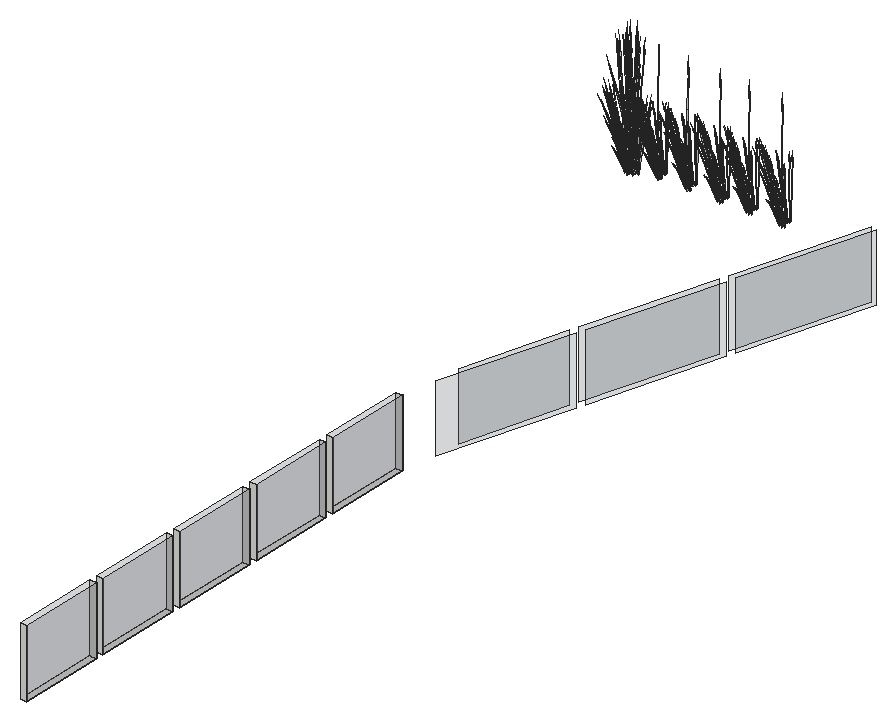
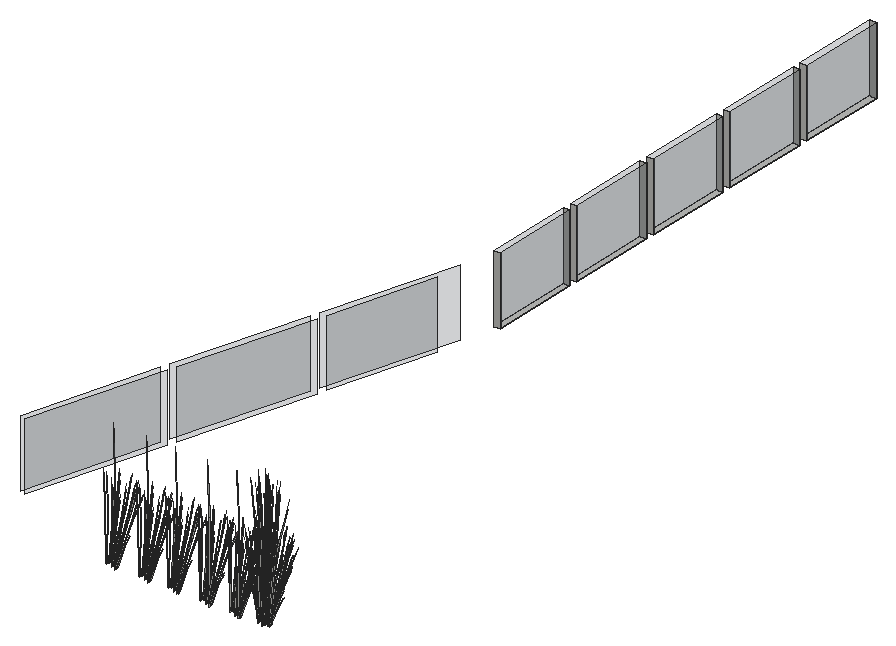
# SketchUp Ruby script. Lengths in inches.
U = 1.inch
M = Sketchup.active_model
def pt(a) = Geom::Point3d.new(a.map { |v| v * U })
def face(e, loops, mat)
  f = e.add_face(loops[0].map { |a| pt(a) })
  loops[1..].each { |l| e.add_face(l.map { |a| pt(a) }).erase! }
  f.material = f.back_material = mat if mat
  f
end
# faces: each face lists its corners as indices into pts; further lists are holes
def faces(e, pts, list, mat = nil) = list.each { |f| face(e, (f[0].is_a?(Array) ? f : [f]).map { |l| l.map { |i| pts[i] } }, mat) }
# xy, xz, yz: faces in a plane at the given z, y or x. An outline is a flat list of corners, or four numbers for a rectangle; further outlines are holes
def ring(l) = l.size == 4 ? [[l[0], l[1]], [l[2], l[1]], [l[2], l[3]], [l[0], l[3]]] : l.each_slice(2).to_a
def flat(e, list, mat, &to3) = list.each { |f| face(e, (f[0].is_a?(Array) ? f : [f]).map { |l| ring(l).map { |u, v| to3.(u, v) } }, mat) }
def xy(e, z, list, mat = nil) = flat(e, list, mat) { |x, y| [x, y, z] }
def xz(e, y, list, mat = nil) = flat(e, list, mat) { |x, z| [x, y, z] }
def yz(e, x, list, mat = nil) = flat(e, list, mat) { |y, z| [x, y, z] }
def lines(e, pts, list) = list.each { |a, b| e.add_line(pt(pts[a]), pt(pts[b])) }
# prism: a flat outline (further loops are holes) pulled along v
def prism(e, loops, v, mat = nil)
  f = face(e, loops, mat); d = Geom::Vector3d.new(v.map { |x| x * U })
  f.pushpull(f.normal.samedirection?(d) ? d.length : -d.length)
end
def box(e, o, s, mat = nil) = prism(e, [[o, [o[0] + s[0], o[1], o[2]], [o[0] + s[0], o[1] + s[1], o[2]], [o[0], o[1] + s[1], o[2]]]], [0, 0, s[2]], mat)
def at(x, y, z, deg = 0) = Geom::Transformation.translation(pt([x, y, z])) * Geom::Transformation.rotation(ORIGIN, Z_AXIS, deg.degrees)
def axes(o, x, y, z) = Geom::Transformation.new([*x, 0, *y, 0, *z, 0, *pt(o).to_a, 1])
def part(name) = M.definitions.add(name)
# library, detail: a bought-in or finely detailed component or shape, given as its bounding box
def library(name, o, s) = part(name).tap { |d| box(d.entities, o, s) }
def detail(e, o, s) = box(e.add_group.entities, o, s)
def put(e, d, t, mat = nil) = e.add_instance(d, t).tap { |i| i.material = mat if mat }
def group(e, t, mat = nil) = e.add_group.tap { |g| g.transformation = t; g.material = mat if mat }.entities
root = M.entities
M.materials.add("Glass_Basic_01").color = [105, 113, 122]
M.materials["Glass_Basic_01"].alpha = 0.25
M.materials.add("LightPink_Translucent").color = [144, 107, 117]
M.materials["LightPink_Translucent"].alpha = 0.75
c1 = part("blade")
p = [[2.15,0.21,22],[0,0.17,0],[0.09,0.45,0],[2.18,0.31,22],[2.29,0.31,22],[0.38,0.45,0],
  [2.48,0.24,33],[2.49,0.24,33],[2.48,0.22,33]]
faces(c1.entities,p,[[0,1,2,3],[4,5,2,3],[6,3,4,7],[8,0,3,6]])
c2 = part("seeds")
p = [[0.3,-0.1,1.38],[-0.01,-0.03,1.59],[-0.01,-0.03,0.03],[0.14,-0.07,-0.07],[0.29,-0.03,3],[0.15,0.01,3.11]]
faces(c2.entities,p,[[0,1,2,3],[1,0,4,5]],"LightPink_Translucent")
c3 = part("blade with seeds")
put(c3.entities,c1,at(0,0,0))
put(c3.entities,c2,axes([2.4,0.25,30.99],[1.5799,-0.05474,1.17369],[-0.12525,1.92788,0.29478],[-0.07173,-0.02425,1.56792]))
xy(root,398,[[300,8,303,49],[300,53,303,94],[300,98,303,139],[300,143,303,184],[300,188,303,229]])
xz(root,8,[[300,398,303,430]])
xz(root,49,[[300,398,303,430]])
xz(root,53,[[300,398,303,430]])
xz(root,94,[[300,398,303,430]])
xz(root,98,[[300,398,303,430]])
xz(root,139,[[300,398,303,430]])
xz(root,143,[[300,398,303,430]])
xz(root,184,[[300,398,303,430]])
xz(root,188,[[300,398,303,430]])
xz(root,229,[[300,398,303,430]])
yz(root,300,[[8,398,49,430],[53,398,94,430],[98,398,139,430],[143,398,184,430],[188,398,229,430]],"Glass_Basic_01")
yz(root,303,[[8,398,49,430],[53,398,94,430],[98,398,139,430],[143,398,184,430],[188,398,229,430]],"Glass_Basic_01")
p = [[323.78,305.43,398],[323.78,305.43,430],[306.07,244.92,430],[306.07,244.92,398],[306.5625,257.28,430],[320.65,305.43,430],
  [320.65,305.43,398],[306.5625,257.28,398],[339.51,369.86,430],[339.51,369.86,398],[321.78,309.27,398],[321.78,309.27,430],
  [324.9,309.27,430],[324.9,309.27,398],[342.64,369.86,398],[342.64,369.86,430],[358.6,435.09,398],[340.64,373.7,398],
  [340.64,373.7,430],[358.6,435.09,430],[361.5,434.3,430],[343.76,373.7,430],[343.76,373.7,398],[361.5,434.3,398]]
faces(root,p,[[0,1,2,3],[4,5,6,7],[8,9,10,11],[12,13,14,15],[16,17,18,19],[20,21,22,23]],"Glass_Basic_01")
put(root,c3,axes([227.93,454.43,399.875],[0.11485,0.17291,1.71376],[-0.53072,0.14557,0.13857],[-0.11995,-0.27145,0.73262]))
put(root,c3,axes([229.99,454.18,398.59],[-0.14282,0.10901,1.43002],[-0.42773,-0.19079,-0.30754],[0.07929,-0.23728,0.61141]))
put(root,c3,axes([229.34,454.56,400.98],[-0.23981,-0.43789,-0.71045],[0.49365,-0.24404,0.08574],[-0.05608,-0.21158,1.00501]))
put(root,c3,axes([227.78,453.97,398.59],[-0.03043,0.17617,1.43002],[-0.4448,0.14748,-0.30754],[-0.10397,-0.22771,0.61141]))
put(root,c3,axes([230.34,454.99,400.98],[0.01307,-0.49815,-0.71045],[0.55054,0.03346,0.08574],[0.0581,-0.21104,1.00501]))
put(root,c3,axes([229.39,454.1875,400.53],[0.15148,-0.41415,-0.35414],[0.44193,0.12079,0.4572],[-0.04052,-0.16674,0.87481]))
put(root,c3,axes([229.72,454.74,399.875],[-0.09355,0.18511,1.71376],[-0.39247,-0.38307,0.13857],[0.17705,-0.23875,0.73262]))
put(root,c3,axes([229.16,454.47,400.68],[-0.49392,-0.135,-0.51099],[0.1693,-0.46287,-0.3958],[-0.04529,-0.18636,0.97773]))
put(root,c3,axes([229.47,453.3125,398.77],[0.06446,0.31404,1.1486],[-0.35756,-0.17393,0.84392],[0.03848,-0.1608,0.25299]))
put(root,c3,axes([230.23,454.82,400.68],[-0.35968,-0.36185,-0.51099],[0.37996,-0.3169,-0.3958],[0.05473,-0.18385,0.97773]))
put(root,c3,axes([230.57,454.6875,400.53],[0.33997,-0.28354,-0.35414],[0.32182,0.32376,0.4572],[0.04897,-0.1645,0.87481]))
put(root,c3,axes([227.63,453.69,398.77],[0.2621,0.18744,1.1486],[-0.38171,0.11267,0.84392],[-0.08167,-0.14405,0.25299]))
put(root,c3,axes([228.26,454.68,400.98],[-0.42844,-0.2603,-0.71045],[0.30448,-0.45614,0.08574],[-0.15523,-0.15542,1.00501]))
put(root,c3,axes([228.11,454.34,400.53],[-0.0776,-0.43378,-0.35414],[0.44361,-0.11454,0.4572],[-0.11915,-0.12431,0.87481]))
put(root,c3,axes([227.16,454.97,399.875],[0.18664,0.09279,1.71376],[-0.38624,0.38925,0.13857],[-0.24072,-0.1756,0.73262]))
put(root,c3,axes([228.06,454.7,400.68],[-0.4958,0.12802,-0.51099],[-0.08673,-0.48481,-0.3958],[-0.13317,-0.13893,0.97773]))
put(root,c3,axes([230.99,455.85,400.98],[0.26246,-0.42493,-0.71045],[0.45991,0.30199,0.08574],[0.15671,-0.15395,1.00501]))
put(root,c3,axes([228.15,454.62,398.375],[-0.31414,-0.53965,0],[0.52557,-0.30095,-0.51607],[0.1197,-0.06854,1.63711]))
put(root,c3,axes([230.97,455.66,400.68],[-0.12908,-0.49174,-0.51099],[0.48882,-0.08602,-0.3958],[0.14008,-0.13208,0.97773]))
put(root,c3,axes([228.84,453.97,398.13],[-0.34721,0.30895,-0.03893],[-0.31814,-0.33837,-0.17649],[-0.0224,-0.09588,0.58215]))
put(root,c3,axes([229.28,457.63,399.33],[0.4342,0.21716,1.51261],[-0.42537,0.46784,0.59816],[-0.19053,-0.27728,1.26806]))
put(root,c3,axes([231.37,455.46,398.59],[-0.1795,-0.01595,1.43002],[-0.18389,-0.42791,-0.30754],[0.22051,-0.12105,0.61141]))
put(root,c3,axes([231.57,454.68,398.77],[-0.16736,0.27414,1.1486],[-0.14385,-0.36832,0.84392],[0.13822,-0.09229,0.25299]))
put(root,c3,axes([231.33,455.71,400.53],[0.43736,-0.07697,-0.35414],[0.11549,0.43998,0.4572],[0.12533,-0.11818,0.87481]))
put(root,c3,axes([227.08,455.1,400.53],[-0.28589,-0.33718,-0.35414],[0.32644,-0.31919,0.4572],[-0.16586,-0.04856,0.87481]))
put(root,c3,axes([227.11,454.53,398.13],[-0.14494,0.43975,-0.03893],[-0.4461,-0.13527,-0.17649],[-0.06773,-0.07192,0.58215]))
put(root,c3,axes([226.875,456.54,398.375],[-0.62828,0,0],[0,-0.6019,-0.51607],[0,-0.13709,1.63711]))
put(root,c3,axes([226.98,455.46,398.59],[0.0981,0.14994,1.43002],[-0.22605,0.40756,-0.30754],[-0.23211,-0.09741,0.61141]))
put(root,c3,axes([239.17,458.68,399.875],[0.11485,0.17291,1.71376],[-0.53072,0.14557,0.13857],[-0.11995,-0.27145,0.73262]))
put(root,c3,axes([252.88,458.68,399.875],[0.11485,0.17291,1.71376],[-0.53072,0.14557,0.13857],[-0.11995,-0.27145,0.73262]))
put(root,c3,axes([268.125,458.68,399.875],[0.11485,0.17291,1.71376],[-0.53072,0.14557,0.13857],[-0.11995,-0.27145,0.73262]))
put(root,c3,axes([281.74,458.68,399.875],[0.11485,0.17291,1.71376],[-0.53072,0.14557,0.13857],[-0.11995,-0.27145,0.73262]))
put(root,c3,axes([297.27,458.68,399.875],[0.11485,0.17291,1.71376],[-0.53072,0.14557,0.13857],[-0.11995,-0.27145,0.73262]))
put(root,c3,axes([227.39,455.33,400.98],[-0.50227,-0.01297,-0.71045],[0.03373,-0.54602,0.08574],[-0.21278,-0.05762,1.00501]))
put(root,c3,axes([241.24,458.43,398.59],[-0.14282,0.10901,1.43002],[-0.42773,-0.19079,-0.30754],[0.07929,-0.23728,0.61141]))
put(root,c3,axes([254.94,458.43,398.59],[-0.14282,0.10901,1.43002],[-0.42773,-0.19079,-0.30754],[0.07929,-0.23728,0.61141]))
put(root,c3,axes([270.19,458.43,398.59],[-0.14282,0.10901,1.43002],[-0.42773,-0.19079,-0.30754],[0.07929,-0.23728,0.61141]))
put(root,c3,axes([283.81,458.43,398.59],[-0.14282,0.10901,1.43002],[-0.42773,-0.19079,-0.30754],[0.07929,-0.23728,0.61141]))
put(root,c3,axes([299.34,458.43,398.59],[-0.14282,0.10901,1.43002],[-0.42773,-0.19079,-0.30754],[0.07929,-0.23728,0.61141]))
put(root,c3,axes([240.58,458.81,400.98],[-0.23981,-0.43789,-0.71045],[0.49365,-0.24404,0.08574],[-0.05608,-0.21158,1.00501]))
put(root,c3,axes([254.29,458.81,400.98],[-0.23981,-0.43789,-0.71045],[0.49365,-0.24404,0.08574],[-0.05608,-0.21158,1.00501]))
put(root,c3,axes([269.54,458.81,400.98],[-0.23981,-0.43789,-0.71045],[0.49365,-0.24404,0.08574],[-0.05608,-0.21158,1.00501]))
put(root,c3,axes([283.15,458.81,400.98],[-0.23981,-0.43789,-0.71045],[0.49365,-0.24404,0.08574],[-0.05608,-0.21158,1.00501]))
put(root,c3,axes([298.68,458.81,400.98],[-0.23981,-0.43789,-0.71045],[0.49365,-0.24404,0.08574],[-0.05608,-0.21158,1.00501]))
put(root,c3,axes([239.02,458.22,398.59],[-0.03043,0.17617,1.43002],[-0.4448,0.14748,-0.30754],[-0.10397,-0.22771,0.61141]))
put(root,c3,axes([252.73,458.22,398.59],[-0.03043,0.17617,1.43002],[-0.4448,0.14748,-0.30754],[-0.10397,-0.22771,0.61141]))
put(root,c3,axes([267.98,458.22,398.59],[-0.03043,0.17617,1.43002],[-0.4448,0.14748,-0.30754],[-0.10397,-0.22771,0.61141]))
put(root,c3,axes([281.59,458.22,398.59],[-0.03043,0.17617,1.43002],[-0.4448,0.14748,-0.30754],[-0.10397,-0.22771,0.61141]))
put(root,c3,axes([297.125,458.22,398.59],[-0.03043,0.17617,1.43002],[-0.4448,0.14748,-0.30754],[-0.10397,-0.22771,0.61141]))
put(root,c3,axes([227.36,456.38,398.33],[-0.46736,0.45277,0.30756],[-0.46764,-0.44801,-0.36492],[-0.01632,-0.12858,1.64885]))
put(root,c3,axes([241.58,459.23,400.98],[0.01307,-0.49815,-0.71045],[0.55054,0.03346,0.08574],[0.0581,-0.21104,1.00501]))
put(root,c3,axes([255.29,459.23,400.98],[0.01307,-0.49815,-0.71045],[0.55054,0.03346,0.08574],[0.0581,-0.21104,1.00501]))
put(root,c3,axes([270.54,459.23,400.98],[0.01307,-0.49815,-0.71045],[0.55054,0.03346,0.08574],[0.0581,-0.21104,1.00501]))
put(root,c3,axes([284.15,459.23,400.98],[0.01307,-0.49815,-0.71045],[0.55054,0.03346,0.08574],[0.0581,-0.21104,1.00501]))
put(root,c3,axes([299.68,459.23,400.98],[0.01307,-0.49815,-0.71045],[0.55054,0.03346,0.08574],[0.0581,-0.21104,1.00501]))
put(root,c3,axes([228.85,456.59,398.43],[0.56613,0.26102,0.24065],[-0.27246,0.54236,0.50002],[0,-0.12502,1.60543]))
put(root,c3,axes([228.625,457.32,398.4375],[0.13317,-0.63814,-0.23429],[0.63143,0.11124,0.51271],[-0.11033,-0.08813,1.5644]))
put(root,c3,axes([240.63,458.43,400.53],[0.15148,-0.41415,-0.35414],[0.44193,0.12079,0.4572],[-0.04052,-0.16674,0.87481]))
put(root,c3,axes([254.34,458.43,400.53],[0.15148,-0.41415,-0.35414],[0.44193,0.12079,0.4572],[-0.04052,-0.16674,0.87481]))
put(root,c3,axes([269.59,458.43,400.53],[0.15148,-0.41415,-0.35414],[0.44193,0.12079,0.4572],[-0.04052,-0.16674,0.87481]))
put(root,c3,axes([283.2,458.43,400.53],[0.15148,-0.41415,-0.35414],[0.44193,0.12079,0.4572],[-0.04052,-0.16674,0.87481]))
put(root,c3,axes([298.73,458.43,400.53],[0.15148,-0.41415,-0.35414],[0.44193,0.12079,0.4572],[-0.04052,-0.16674,0.87481]))
put(root,c3,axes([240.96,458.98,399.875],[-0.09355,0.18511,1.71376],[-0.39247,-0.38307,0.13857],[0.17705,-0.23875,0.73262]))
put(root,c3,axes([254.67,458.98,399.875],[-0.09355,0.18511,1.71376],[-0.39247,-0.38307,0.13857],[0.17705,-0.23875,0.73262]))
put(root,c3,axes([269.92,458.98,399.875],[-0.09355,0.18511,1.71376],[-0.39247,-0.38307,0.13857],[0.17705,-0.23875,0.73262]))
put(root,c3,axes([283.53,458.98,399.875],[-0.09355,0.18511,1.71376],[-0.39247,-0.38307,0.13857],[0.17705,-0.23875,0.73262]))
put(root,c3,axes([299.0625,458.98,399.875],[-0.09355,0.18511,1.71376],[-0.39247,-0.38307,0.13857],[0.17705,-0.23875,0.73262]))
put(root,c3,axes([227.22,455.4375,400.68],[-0.36484,0.35674,-0.51099],[-0.31952,-0.37685,-0.3958],[-0.18537,-0.05428,0.97773]))
put(root,c3,axes([226.4,455.91,398.77],[0.32078,-0.03854,1.1486],[-0.20348,0.33954,0.84392],[-0.15852,-0.05093,0.25299]))
put(root,c3,axes([240.4,458.72,400.68],[-0.49392,-0.135,-0.51099],[0.1693,-0.46287,-0.3958],[-0.04529,-0.18636,0.97773]))
put(root,c3,axes([254.11,458.72,400.68],[-0.49392,-0.135,-0.51099],[0.1693,-0.46287,-0.3958],[-0.04529,-0.18636,0.97773]))
put(root,c3,axes([269.36,458.72,400.68],[-0.49392,-0.135,-0.51099],[0.1693,-0.46287,-0.3958],[-0.04529,-0.18636,0.97773]))
put(root,c3,axes([282.97,458.72,400.68],[-0.49392,-0.135,-0.51099],[0.1693,-0.46287,-0.3958],[-0.04529,-0.18636,0.97773]))
put(root,c3,axes([298.5,458.72,400.68],[-0.49392,-0.135,-0.51099],[0.1693,-0.46287,-0.3958],[-0.04529,-0.18636,0.97773]))
put(root,c3,axes([240.71,457.56,398.77],[0.06446,0.31404,1.1486],[-0.35756,-0.17393,0.84392],[0.03848,-0.1608,0.25299]))
put(root,c3,axes([254.42,457.56,398.77],[0.06446,0.31404,1.1486],[-0.35756,-0.17393,0.84392],[0.03848,-0.1608,0.25299]))
put(root,c3,axes([269.67,457.56,398.77],[0.06446,0.31404,1.1486],[-0.35756,-0.17393,0.84392],[0.03848,-0.1608,0.25299]))
put(root,c3,axes([283.28,457.56,398.77],[0.06446,0.31404,1.1486],[-0.35756,-0.17393,0.84392],[0.03848,-0.1608,0.25299]))
put(root,c3,axes([298.81,457.56,398.77],[0.06446,0.31404,1.1486],[-0.35756,-0.17393,0.84392],[0.03848,-0.1608,0.25299]))
put(root,c3,axes([228.66,456.22,398.72],[-0.54562,0.03324,0.44739],[-0.04934,-0.55185,-0.21531],[0.09768,-0.05593,1.43643]))
put(root,c3,axes([241.47,459.07,400.68],[-0.35968,-0.36185,-0.51099],[0.37996,-0.3169,-0.3958],[0.05473,-0.18385,0.97773]))
put(root,c3,axes([255.18,459.07,400.68],[-0.35968,-0.36185,-0.51099],[0.37996,-0.3169,-0.3958],[0.05473,-0.18385,0.97773]))
put(root,c3,axes([270.43,459.07,400.68],[-0.35968,-0.36185,-0.51099],[0.37996,-0.3169,-0.3958],[0.05473,-0.18385,0.97773]))
put(root,c3,axes([284.04,459.07,400.68],[-0.35968,-0.36185,-0.51099],[0.37996,-0.3169,-0.3958],[0.05473,-0.18385,0.97773]))
put(root,c3,axes([299.57,459.07,400.68],[-0.35968,-0.36185,-0.51099],[0.37996,-0.3169,-0.3958],[0.05473,-0.18385,0.97773]))
put(root,c3,axes([227.26,456.63,398.48],[0,0.53854,0.49651],[-0.56215,0,0],[0,-0.12266,1.57504]))
put(root,c3,axes([231.2,456.75,400.68],[0.13612,-0.48987,-0.51099],[0.46669,0.16791,-0.3958],[0.1879,-0.04492,0.97773]))
put(root,c3,axes([230.46,454.75,398.375],[0.31414,-0.53965,0],[0.52557,0.30095,-0.51607],[0.1197,0.06854,1.63711]))
put(root,c3,axes([226.76,455.82,399.875],[0.20841,-0.0122,1.71376],[-0.13825,0.52864,0.13857],[-0.297,-0.0327,0.73262]))
put(root,c3,axes([228.65,456.42,398.36],[0.21845,0.6022,0.45755],[-0.62418,0.20941,0.17955],[0.00763,-0.11065,1.58856]))
put(root,c3,axes([231.7,456.89,397.98],[-0.32361,0.06463,1.41583],[-0.05151,-0.51444,0.08104],[0.22666,-0.07786,0.80566]))
put(root,c3,axes([232.29,456.43,398.26],[-0.31151,-0.34437,-0.06488],[0.34117,-0.31553,-0.29416],[0.09667,-0.02221,0.97024]))
put(root,c3,axes([228.54,456.9,398.72],[-0.24378,0.48527,0.44739],[-0.50654,-0.23354,-0.21531],[0,-0.11186,1.43643]))
put(root,c3,axes([229.43,456.47,398.21],[0,-0.62313,0],[0.62828,0,0],[0,0,1.79456]))
put(root,c3,axes([241.81,458.93,400.53],[0.33997,-0.28354,-0.35414],[0.32182,0.32376,0.4572],[0.04897,-0.1645,0.87481]))
put(root,c3,axes([255.52,458.93,400.53],[0.33997,-0.28354,-0.35414],[0.32182,0.32376,0.4572],[0.04897,-0.1645,0.87481]))
put(root,c3,axes([270.77,458.93,400.53],[0.33997,-0.28354,-0.35414],[0.32182,0.32376,0.4572],[0.04897,-0.1645,0.87481]))
put(root,c3,axes([284.38,458.93,400.53],[0.33997,-0.28354,-0.35414],[0.32182,0.32376,0.4572],[0.04897,-0.1645,0.87481]))
put(root,c3,axes([299.91,458.93,400.53],[0.33997,-0.28354,-0.35414],[0.32182,0.32376,0.4572],[0.04897,-0.1645,0.87481]))
put(root,c3,axes([238.87,457.9375,398.77],[0.2621,0.18744,1.1486],[-0.38171,0.11267,0.84392],[-0.08167,-0.14405,0.25299]))
put(root,c3,axes([252.58,457.9375,398.77],[0.2621,0.18744,1.1486],[-0.38171,0.11267,0.84392],[-0.08167,-0.14405,0.25299]))
put(root,c3,axes([267.83,457.9375,398.77],[0.2621,0.18744,1.1486],[-0.38171,0.11267,0.84392],[-0.08167,-0.14405,0.25299]))
put(root,c3,axes([281.44,457.9375,398.77],[0.2621,0.18744,1.1486],[-0.38171,0.11267,0.84392],[-0.08167,-0.14405,0.25299]))
put(root,c3,axes([296.97,457.9375,398.77],[0.2621,0.18744,1.1486],[-0.38171,0.11267,0.84392],[-0.08167,-0.14405,0.25299]))
put(root,c3,axes([239.5,458.93,400.98],[-0.42844,-0.2603,-0.71045],[0.30448,-0.45614,0.08574],[-0.15523,-0.15542,1.00501]))
put(root,c3,axes([253.21,458.93,400.98],[-0.42844,-0.2603,-0.71045],[0.30448,-0.45614,0.08574],[-0.15523,-0.15542,1.00501]))
put(root,c3,axes([268.46,458.93,400.98],[-0.42844,-0.2603,-0.71045],[0.30448,-0.45614,0.08574],[-0.15523,-0.15542,1.00501]))
put(root,c3,axes([282.07,458.93,400.98],[-0.42844,-0.2603,-0.71045],[0.30448,-0.45614,0.08574],[-0.15523,-0.15542,1.00501]))
put(root,c3,axes([297.6,458.93,400.98],[-0.42844,-0.2603,-0.71045],[0.30448,-0.45614,0.08574],[-0.15523,-0.15542,1.00501]))
put(root,c3,axes([230.19,455.03,398.48],[-0.47024,-0.26927,0.49651],[0.28107,-0.48284,0],[0.1071,0.06133,1.57504]))
put(root,c3,axes([231.11,456.93,400.98],[0.44151,-0.23785,-0.71045],[0.24605,0.4896,0.08574],[0.21333,-0.05562,1.00501]))
put(root,c3,axes([239.36,458.59,400.53],[-0.0776,-0.43378,-0.35414],[0.44361,-0.11454,0.4572],[-0.11915,-0.12431,0.87481]))
put(root,c3,axes([253.0625,458.59,400.53],[-0.0776,-0.43378,-0.35414],[0.44361,-0.11454,0.4572],[-0.11915,-0.12431,0.87481]))
put(root,c3,axes([268.3125,458.59,400.53],[-0.0776,-0.43378,-0.35414],[0.44361,-0.11454,0.4572],[-0.11915,-0.12431,0.87481]))
put(root,c3,axes([281.93,458.59,400.53],[-0.0776,-0.43378,-0.35414],[0.44361,-0.11454,0.4572],[-0.11915,-0.12431,0.87481]))
put(root,c3,axes([297.46,458.59,400.53],[-0.0776,-0.43378,-0.35414],[0.44361,-0.11454,0.4572],[-0.11915,-0.12431,0.87481]))
put(root,c3,axes([229.13,456.08,398.36],[-0.4166,0.48873,0.45755],[-0.49494,-0.43142,0.17955],[0.10044,-0.04877,1.58856]))
put(root,c3,axes([229.59,456.96,398.3],[-0.46736,-0.46353,-0.06131],[0.46764,-0.46381,0],[-0.01632,-0.01619,1.75571]))
put(root,c3,axes([228.41,455.28,398.47],[-0.14515,0.53522,0.17642],[-0.53115,-0.15146,0.35086],[0.09175,-0.00261,1.60407]))
put(root,c3,axes([229.52,455.87,398.62],[0.09693,-0.48062,0.1448],[0.47357,0.08343,-0.41347],[0.08619,0.04935,1.26744]))
put(root,c3,axes([228.7,457.01,398.36],[0.63506,0.11347,0.45755],[-0.12924,0.64083,0.17955],[-0.09281,-0.06188,1.58856]))
put(root,c3,axes([238.4,459.22,399.875],[0.18664,0.09279,1.71376],[-0.38624,0.38925,0.13857],[-0.24072,-0.1756,0.73262]))
put(root,c3,axes([252.11,459.22,399.875],[0.18664,0.09279,1.71376],[-0.38624,0.38925,0.13857],[-0.24072,-0.1756,0.73262]))
put(root,c3,axes([267.36,459.22,399.875],[0.18664,0.09279,1.71376],[-0.38624,0.38925,0.13857],[-0.24072,-0.1756,0.73262]))
put(root,c3,axes([280.97,459.22,399.875],[0.18664,0.09279,1.71376],[-0.38624,0.38925,0.13857],[-0.24072,-0.1756,0.73262]))
put(root,c3,axes([296.5,459.22,399.875],[0.18664,0.09279,1.71376],[-0.38624,0.38925,0.13857],[-0.24072,-0.1756,0.73262]))
put(root,c3,axes([229.32,456,398.72],[-0.30184,-0.45202,0.44739],[0.45719,-0.31831,-0.21531],[0.09768,0.05593,1.43643]))
put(root,c3,axes([239.3,458.94,400.68],[-0.4958,0.12802,-0.51099],[-0.08673,-0.48481,-0.3958],[-0.13317,-0.13893,0.97773]))
put(root,c3,axes([253.01,458.94,400.68],[-0.4958,0.12802,-0.51099],[-0.08673,-0.48481,-0.3958],[-0.13317,-0.13893,0.97773]))
put(root,c3,axes([268.26,458.94,400.68],[-0.4958,0.12802,-0.51099],[-0.08673,-0.48481,-0.3958],[-0.13317,-0.13893,0.97773]))
put(root,c3,axes([281.875,458.94,400.68],[-0.4958,0.12802,-0.51099],[-0.08673,-0.48481,-0.3958],[-0.13317,-0.13893,0.97773]))
put(root,c3,axes([297.4,458.94,400.68],[-0.4958,0.12802,-0.51099],[-0.08673,-0.48481,-0.3958],[-0.13317,-0.13893,0.97773]))
put(root,c3,axes([228.36,458.04,398.47],[0.53992,-0.14294,0.17642],[0.13332,0.53195,0.35086],[-0.04815,-0.07751,1.60407]))
put(root,c3,axes([231.49,456.97,400.53],[0.41757,0.15024,-0.35414],[-0.12179,0.4383,0.4572],[0.16812,-0.04019,0.87481]))
put(root,c3,axes([226.58,456.27,400.53],[-0.41757,-0.15024,-0.35414],[0.12179,-0.4383,0.4572],[-0.16812,0.04019,0.87481]))
put(root,c3,axes([229.86,456.61,398.21],[0.56215,0,0],[0,0.55754,0],[0,0,1.78407]))
put(root,c3,axes([242.23,460.1,400.98],[0.26246,-0.42493,-0.71045],[0.45991,0.30199,0.08574],[0.15671,-0.15395,1.00501]))
put(root,c3,axes([255.94,460.1,400.98],[0.26246,-0.42493,-0.71045],[0.45991,0.30199,0.08574],[0.15671,-0.15395,1.00501]))
put(root,c3,axes([271.1875,460.1,400.98],[0.26246,-0.42493,-0.71045],[0.45991,0.30199,0.08574],[0.15671,-0.15395,1.00501]))
put(root,c3,axes([284.8,460.1,400.98],[0.26246,-0.42493,-0.71045],[0.45991,0.30199,0.08574],[0.15671,-0.15395,1.00501]))
put(root,c3,axes([300.33,460.1,400.98],[0.26246,-0.42493,-0.71045],[0.45991,0.30199,0.08574],[0.15671,-0.15395,1.00501]))
put(root,c3,axes([239.39,458.86,398.375],[-0.31414,-0.53965,0],[0.52557,-0.30095,-0.51607],[0.1197,-0.06854,1.63711]))
put(root,c3,axes([253.1,458.86,398.375],[-0.31414,-0.53965,0],[0.52557,-0.30095,-0.51607],[0.1197,-0.06854,1.63711]))
put(root,c3,axes([268.35,458.86,398.375],[-0.31414,-0.53965,0],[0.52557,-0.30095,-0.51607],[0.1197,-0.06854,1.63711]))
put(root,c3,axes([281.96,458.86,398.375],[-0.31414,-0.53965,0],[0.52557,-0.30095,-0.51607],[0.1197,-0.06854,1.63711]))
put(root,c3,axes([297.49,458.86,398.375],[-0.31414,-0.53965,0],[0.52557,-0.30095,-0.51607],[0.1197,-0.06854,1.63711]))
put(root,c3,axes([242.22,459.9,400.68],[-0.12908,-0.49174,-0.51099],[0.48882,-0.08602,-0.3958],[0.14008,-0.13208,0.97773]))
put(root,c3,axes([255.93,459.9,400.68],[-0.12908,-0.49174,-0.51099],[0.48882,-0.08602,-0.3958],[0.14008,-0.13208,0.97773]))
put(root,c3,axes([271.17,459.9,400.68],[-0.12908,-0.49174,-0.51099],[0.48882,-0.08602,-0.3958],[0.14008,-0.13208,0.97773]))
put(root,c3,axes([284.79,459.9,400.68],[-0.12908,-0.49174,-0.51099],[0.48882,-0.08602,-0.3958],[0.14008,-0.13208,0.97773]))
put(root,c3,axes([300.32,459.9,400.68],[-0.12908,-0.49174,-0.51099],[0.48882,-0.08602,-0.3958],[0.14008,-0.13208,0.97773]))
put(root,c3,axes([230.02,455.31,398.47],[-0.53992,0.14294,0.17642],[-0.13332,-0.53195,0.35086],[0.04815,0.07751,1.60407]))
put(root,c3,axes([240.08,458.21,398.13],[-0.34721,0.30895,-0.03893],[-0.31814,-0.33837,-0.17649],[-0.0224,-0.09588,0.58215]))
put(root,c3,axes([253.79,458.21,398.13],[-0.34721,0.30895,-0.03893],[-0.31814,-0.33837,-0.17649],[-0.0224,-0.09588,0.58215]))
put(root,c3,axes([269.04,458.21,398.13],[-0.34721,0.30895,-0.03893],[-0.31814,-0.33837,-0.17649],[-0.0224,-0.09588,0.58215]))
put(root,c3,axes([282.65,458.21,398.13],[-0.34721,0.30895,-0.03893],[-0.31814,-0.33837,-0.17649],[-0.0224,-0.09588,0.58215]))
put(root,c3,axes([298.18,458.21,398.13],[-0.34721,0.30895,-0.03893],[-0.31814,-0.33837,-0.17649],[-0.0224,-0.09588,0.58215]))
